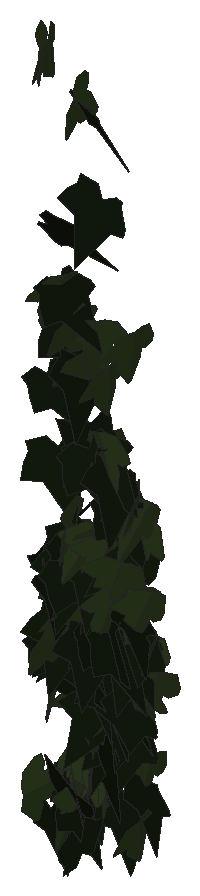
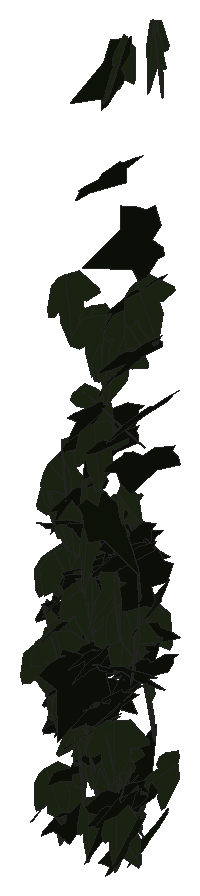
# SketchUp Ruby script. Lengths in inches.
U = 1.inch
M = Sketchup.active_model
def pt(a) = Geom::Point3d.new(a.map { |v| v * U })
def face(e, loops, mat)
  f = e.add_face(loops[0].map { |a| pt(a) })
  loops[1..].each { |l| e.add_face(l.map { |a| pt(a) }).erase! }
  f.material = f.back_material = mat if mat
  f
end
# faces: each face lists its corners as indices into pts; further lists are holes
def faces(e, pts, list, mat = nil) = list.each { |f| face(e, (f[0].is_a?(Array) ? f : [f]).map { |l| l.map { |i| pts[i] } }, mat) }
# xy, xz, yz: faces in a plane at the given z, y or x. An outline is a flat list of corners, or four numbers for a rectangle; further outlines are holes
def ring(l) = l.size == 4 ? [[l[0], l[1]], [l[2], l[1]], [l[2], l[3]], [l[0], l[3]]] : l.each_slice(2).to_a
def flat(e, list, mat, &to3) = list.each { |f| face(e, (f[0].is_a?(Array) ? f : [f]).map { |l| ring(l).map { |u, v| to3.(u, v) } }, mat) }
def xy(e, z, list, mat = nil) = flat(e, list, mat) { |x, y| [x, y, z] }
def xz(e, y, list, mat = nil) = flat(e, list, mat) { |x, z| [x, y, z] }
def yz(e, x, list, mat = nil) = flat(e, list, mat) { |y, z| [x, y, z] }
def lines(e, pts, list) = list.each { |a, b| e.add_line(pt(pts[a]), pt(pts[b])) }
# prism: a flat outline (further loops are holes) pulled along v
def prism(e, loops, v, mat = nil)
  f = face(e, loops, mat); d = Geom::Vector3d.new(v.map { |x| x * U })
  f.pushpull(f.normal.samedirection?(d) ? d.length : -d.length)
end
def box(e, o, s, mat = nil) = prism(e, [[o, [o[0] + s[0], o[1], o[2]], [o[0] + s[0], o[1] + s[1], o[2]], [o[0], o[1] + s[1], o[2]]]], [0, 0, s[2]], mat)
def at(x, y, z, deg = 0) = Geom::Transformation.translation(pt([x, y, z])) * Geom::Transformation.rotation(ORIGIN, Z_AXIS, deg.degrees)
def axes(o, x, y, z) = Geom::Transformation.new([*x, 0, *y, 0, *z, 0, *pt(o).to_a, 1])
def part(name) = M.definitions.add(name)
# library, detail: a bought-in or finely detailed component or shape, given as its bounding box
def library(name, o, s) = part(name).tap { |d| box(d.entities, o, s) }
def detail(e, o, s) = box(e.add_group.entities, o, s)
def put(e, d, t, mat = nil) = e.add_instance(d, t).tap { |i| i.material = mat if mat }
def group(e, t, mat = nil) = e.add_group.tap { |g| g.transformation = t; g.material = mat if mat }.entities
root = M.entities
M.materials.add("efeu1").color = [18, 25, 13]
M.materials.add("efeu2").color = [43, 57, 29]
c1 = part("ivyleaf_10")
p = [[0,0.5,-0.03],[-0.0625,2.02,-0.43],[-0.19,2.01,-0.46],[-0.54,1.05,-0.29],[-0.52,0.625,-0.18],[-0.83,0.76,-0.28],
  [-1.16,0.64,-0.33],[-1.15,0.33,-0.24],[-0.77,-0.39,0.02],[-0.3,-0.51,0.16],[0.04,-0.48,0.23],[-0.02,2.01,-0.4375],
  [-0.06,2.01,-0.43],[0.04,-0.49,0.23],[0.67,-0.49,0.14],[1.38,0.36,-0.2],[1.375,0.51,-0.24],[0.81,0.65,-0.19],
  [0.62,0.59,-0.15],[0.6,1.09,-0.28],[0.5,1.23,-0.31]]
faces(c1.entities,p,[[0,1,2,3,4,5,6,7,8,9,10],[11,12,0,13,14,15,16,17,18,19,20]],"efeu2")
c2 = part("ivyleaf_9")
p = [[1.54,2.16,1.25],[1.36,2.04,1.19],[-0.21,0.99,0.68],[-0.71,1.11,0.82],[-0.85,0.86,0.67],[-0.8,0.17,0.21],
  [-0.9,-0.01,0.1],[-0.67,-0.16,-0.02],[-0.08,-0.08,-0.05],[-0.03,-0.6,-0.4],[0.65,-0.88,-0.66],[0.83,-0.6,-0.49],
  [1.29,-0.42,-0.43],[1.8125,-0.07,-0.26],[1.21,0.44,0.15]]
faces(c2.entities,p,[[0,1,2,3,4,5,6,7,8,9,10,11,12,13,14]],"efeu1")
put(root,c1,axes([531.31,133.06,214.31],[0.38555,-0.60356,-0.56134],[-0.07276,0.59238,-0.68691],[0.82103,0.33592,0.20273]))
put(root,c2,axes([530.73,134.37,206.68],[0.50004,-0.69895,0.12172],[0.07493,-0.09605,-0.85939],[0.7055,0.5056,0.00501]))
put(root,c1,axes([531.26,132.02,237.24],[0.60567,-0.73019,-0.20182],[-0.01894,0.24371,-0.93861],[0.75733,0.59006,0.13793]))
put(root,c2,axes([530.76,133.04,223.34],[0.41024,-0.76261,-0.33412],[0.09273,0.41201,-0.82653],[0.82741,0.33193,0.25829]))
put(root,c1,axes([531.36,134.16,207.32],[-0.0306,-0.83738,-0.23344],[0.00435,0.23343,-0.83793],[0.8693,-0.03064,-0.00402]))
put(root,c1,axes([531.46,132.7,227.38],[-0.14113,-0.90335,0.18428],[-0.04904,-0.1788,-0.91408],[0.92065,-0.148,-0.02045]))
put(root,c2,axes([531.56,134.07,213.17],[-0.80351,-0.35056,0.01012],[0.09038,-0.23142,-0.84077],[0.33887,-0.76953,0.24824]))
put(root,c2,axes([530.95,132.92,213.08],[0.22478,-0.6736,-0.50792],[0.09563,0.54259,-0.67727],[0.8382,0.11874,0.21347]))
put(root,c1,axes([531.56,133.4,215.02],[-0.35311,-0.7704,0.22773],[-0.04685,-0.22858,-0.84594],[0.80199,-0.35255,0.05085]))
put(root,c1,axes([531.44,133.86,206.71],[0.07082,-0.76777,0.36554],[0.05311,-0.36209,-0.77083],[0.84869,0.08672,0.01774]))
put(root,c2,axes([530.98,132.84,206.17],[0.32279,-0.7566,0.18108],[0.0695,-0.16722,-0.82258],[0.77486,0.33018,-0.00166]))
put(root,c1,axes([531.56,134.09,210.61],[-0.51691,-0.71114,-0.02205],[0.06157,-0.01756,-0.8771],[0.70881,-0.51708,0.06011]))
put(root,c2,axes([531.27,134.17,207.89],[0.36615,-0.5321,-0.55869],[-0.27836,0.48566,-0.64497],[0.71957,0.45862,0.03479]))
put(root,c1,axes([531.55,131.9,237.3],[0.26569,-0.83161,-0.43011],[0.00191,0.44757,-0.8642],[0.93626,0.23508,0.12382]))
put(root,c1,axes([531.6,132.23,211.63],[0.48606,-0.70274,-0.28183],[-0.12268,0.25739,-0.85336],[0.74714,0.49943,0.04323]))
put(root,c1,axes([531.4,131.21,207.92],[0.0765,-0.10269,-0.94407],[0.27818,0.908,-0.07622],[0.90798,-0.26954,0.1029]))
put(root,c1,axes([531.65,133.45,214.53],[-0.57947,-0.65111,-0.09346],[0.05323,0.07773,-0.87155],[0.65563,-0.58179,-0.01185]))
put(root,c1,axes([531.52,134.33,210.18],[0.48114,-0.71154,0.07292],[0.07994,-0.03383,-0.85765],[0.71078,0.48545,0.0471]))
put(root,c2,axes([531.17,132.9375,214.83],[0.05217,-0.67786,0.55598],[0.18506,-0.5359,-0.67074],[0.85695,0.15699,0.111]))
put(root,c1,axes([531.84,133.61,215.99],[0.38725,-0.53266,-0.59096],[-0.25962,0.53666,-0.65385],[0.75204,0.45956,0.07859]))
put(root,c1,axes([531.82,132.46,215.96],[0.47407,-0.73454,-0.50008],[-0.14605,0.49468,-0.86507],[0.87653,0.4797,0.12632]))
put(root,c1,axes([531.79,132.96,214.22],[-0.43697,-0.74668,-0.15234],[0.05657,0.14334,-0.86483],[0.75996,-0.44001,-0.02322]))
put(root,c1,axes([531.94,133.71,215.85],[-0.01054,0.17131,0.86807],[-0.36442,0.79024,-0.16038],[-0.80628,-0.35941,0.06114]))
put(root,c2,axes([531.38,133.27,225.4],[0.14211,-0.86458,-0.27161],[0.08904,0.28692,-0.86673],[0.90186,0.10791,0.12837]))
put(root,c2,axes([531.2,132.65,216.01],[0.23828,-0.06865,0.85647],[0.8442,0.18414,-0.22011],[-0.15993,0.86972,0.11421]))
put(root,c2,axes([531.78,132.79,214.02],[-0.5604,-0.68176,-0.20575],[0.1371,0.15363,-0.88249],[0.69881,-0.57687,0.00814]))
put(root,c2,axes([531.1875,132.64,229.65],[0.88444,-0.09046,0.31445],[0.31285,-0.03169,-0.88905],[0.09585,0.93814,0.00029]))
put(root,c2,axes([531.54,132.54,220.9],[-0.14463,-0.80789,-0.42978],[0.15271,0.4077,-0.81778],[0.90226,-0.19851,0.06952]))
put(root,c1,axes([531.9375,131.45,213.97],[-0.20913,-0.61059,-0.74498],[0.20884,0.71546,-0.64502],[0.94032,-0.2947,-0.02244]))
put(root,c2,axes([531.66,133.3,217.22],[0.03492,-0.84123,-0.33092],[0.06151,0.33261,-0.83904],[0.90188,0.00988,0.07004]))
put(root,c1,axes([532.0625,133.6,215.53],[-0.36583,-0.70571,0.40923],[0.10244,-0.48469,-0.74425],[0.80932,-0.25765,0.27918]))
put(root,c2,axes([531.62,132.61,227.42],[0.36174,-0.74749,-0.4514],[-0.0321,0.47689,-0.81542],[0.87263,0.32741,0.15713]))
put(root,c1,axes([532.06,132.68,226],[-0.23724,-0.75455,-0.51758],[0.14702,0.49632,-0.79094],[0.90312,-0.27901,-0.0072]))
put(root,c2,axes([531.83,133.65,207.43],[-0.05794,-0.83191,-0.14877],[0.00108,0.14905,-0.83388],[0.84511,-0.05722,-0.00913]))
put(root,c2,axes([532.51,133.66,218.99],[-0.46241,0.71726,-0.27291],[0.01946,-0.30756,-0.84131],[-0.76718,-0.44013,0.14315]))
put(root,c1,axes([532.75,132.52,214.16],[0.23584,0.0086,-0.88225],[-0.84813,0.25387,-0.22425],[0.24313,0.87723,0.07355]))
put(root,c2,axes([531.89,133.55,207.86],[-0.03088,-0.80519,-0.39924],[0.02736,0.39845,-0.80571],[0.89832,-0.03982,0.01082]))
put(root,c1,axes([532.07,132.8125,208.02],[-0.38647,0.73817,-0.21038],[0.09403,-0.18824,-0.83321],[-0.76179,-0.39772,0.00389]))
put(root,c2,axes([531.84,133.35,211.45],[0.14551,-0.82173,0.2304],[0.15707,-0.20395,-0.82658],[0.83884,0.18073,0.11481]))
put(root,c2,axes([532.32,132.33,207.1875],[0.67125,-0.44023,0.40048],[-0.33428,0.22055,0.80274],[-0.49239,-0.74988,0.00098]))
put(root,c2,axes([532.13,132.49,217.6],[0.18109,-0.52398,-0.70922],[-0.2471,0.66485,-0.5543],[0.84645,0.30619,-0.01009]))
put(root,c2,axes([532.22,134.11,211.43],[-0.20707,-0.85297,0.01207],[0.00344,-0.01326,-0.87772],[0.85305,-0.20699,0.00647]))
put(root,c2,axes([532.39,132.67,216.77],[-0.55726,-0.73513,-0.12476],[0.05694,0.11335,-0.92218],[0.74346,-0.55969,-0.02289]))
put(root,c1,axes([532.5,134.25,207.3],[0.07736,-0.82771,-0.20258],[0.03896,0.20663,-0.8294],[0.85125,0.06577,0.05637]))
put(root,c2,axes([532.16,134.15,213.53],[0.16524,-0.85872,0.01341],[-0.00032,-0.01372,-0.87447],[0.85882,0.16522,-0.00291]))
put(root,c1,axes([532.5625,134.65,209.65],[0.42235,-0.71185,-0.2197],[-0.02377,0.23955,-0.82185],[0.74461,0.41142,0.09839]))
put(root,c1,axes([532.58,132.61,224.8125],[-0.31543,-0.8219,-0.31637],[0.10356,0.29911,-0.88029],[0.87458,-0.33184,-0.00987]))
put(root,c1,axes([532.5,132.96,208.97],[0.57246,0.61048,-0.20411],[-0.11839,-0.16864,-0.83642],[-0.63272,0.58389,-0.02817]))
put(root,c1,axes([532.43,132.39,218.8125],[0.29086,-0.66861,0.59019],[0.30293,-0.5098,-0.72684],[0.8388,0.41596,0.05785]))
put(root,c1,axes([532.51,132.35,207.46],[0.05009,-0.70202,0.61785],[0.24348,-0.58761,-0.6874],[0.90293,0.1974,0.15108]))
put(root,c1,axes([532.72,134.07,217.875],[0.16388,-0.73005,-0.46171],[-0.03906,0.4632,-0.74628],[0.86292,0.15962,0.05391]))
put(root,c1,axes([533,133.49,216.74],[-0.43486,-0.4296,0.66141],[-0.34127,-0.57841,-0.60007],[0.71101,-0.54037,0.11649]))
put(root,c1,axes([532.74,133.21,225.81],[-0.77789,-0.48788,-0.031],[0.04364,-0.01127,-0.91764],[0.48691,-0.77842,0.03272]))
put(root,c1,axes([532.74,133.75,216.09],[0.19134,-0.81308,-0.32498],[-0.02485,0.32747,-0.83395],[0.87527,0.18705,0.04737]))
put(root,c2,axes([532.38,132.71,224.16],[0.08598,-0.89241,0.28531],[0.00142,-0.28638,-0.8962],[0.93691,0.08233,-0.02483]))
put(root,c1,axes([532.9,133.5,208.9375],[-0.46583,-0.6684,0.35346],[-0.08055,-0.36892,-0.80381],[0.7518,-0.45369,0.13288]))
put(root,c2,axes([533.43,132.08,221.72],[-0.28187,0.57149,0.64541],[-0.54893,0.40459,-0.59799],[-0.6647,-0.57647,0.22015]))
put(root,c2,axes([532.81,134.16,212.62],[0.49202,0.72434,-0.01563],[-0.02514,-0.00181,-0.87542],[-0.72407,0.49226,0.01978]))
put(root,c2,axes([532.47,132.32,207.32],[0.31689,-0.74652,-0.26021],[-0.06764,0.25371,-0.81023],[0.78767,0.32212,0.03511]))
put(root,c1,axes([532.98,133.82,209.83],[0.02079,-0.8764,-0.02765],[-0.00126,0.02762,-0.87664],[0.87683,0.02082,-0.0006]))
put(root,c1,axes([532.78,133.89,210.15],[0.37943,-0.75077,0.22454],[0.21086,-0.14246,-0.83264],[0.75473,0.41724,0.11974]))
put(root,c2,axes([532.49,131.89,216.96],[0.37475,-0.6045,-0.70261],[-0.04981,0.74364,-0.66637],[0.92553,0.28479,0.24863]))
put(root,c1,axes([532.72,133.05,208.88],[0.74599,0.41479,0.1404],[0.12893,0.05701,-0.85346],[-0.4185,0.75694,-0.01266]))
put(root,c1,axes([533.07,132.53,218.01],[-0.30655,-0.82735,-0.13894],[0.02839,0.13762,-0.88207],[0.83846,-0.30715,-0.02094]))
put(root,c1,axes([533.09,132.4,218.02],[-0.23874,-0.63954,0.58],[-0.01364,-0.59889,-0.666],[0.86326,-0.18634,0.14988]))
put(root,c1,axes([533.14,133.8,215.49],[-0.4578,-0.74486,0.14939],[-0.0223,-0.16117,-0.87192],[0.75936,-0.45378,0.06446]))
put(root,c2,axes([533.44,131.48,206.12],[-0.75804,0.34514,-0.36247],[-0.33782,0.13257,0.83272],[0.3693,0.82972,0.01772]))
put(root,c1,axes([533.11,133.16,221.39],[-0.20642,-0.8997,-0.06173],[0.00489,0.06221,-0.92303],[0.9018,-0.20627,-0.00913]))
put(root,c2,axes([532.68,133.49,213.23],[0.05114,-0.86786,-0.22976],[0.03693,0.23197,-0.86799],[0.897,0.03993,0.04883]))
put(root,c2,axes([533.04,133.79,216.23],[-0.573,-0.68403,0.03057],[0.02745,-0.06278,-0.89021],[0.68416,-0.57038,0.06132]))
put(root,c2,axes([532.97,134.64,209.03],[-0.30943,-0.78496,0.11855],[0.00926,-0.1308,-0.84188],[0.79381,-0.30446,0.05603]))
put(root,c2,axes([532.97,132.76,213.75],[-0.31182,-0.81495,-0.1063],[0.01122,0.10946,-0.87211],[0.82178,-0.31073,-0.02843]))
put(root,c2,axes([532.6875,133.4,217.67],[-0.32571,-0.45171,-0.70705],[0.64127,0.35507,-0.52225],[0.54105,-0.69277,0.19335]))
put(root,c1,axes([533.17,131.48,235.84],[0.12046,-0.59248,-0.75944],[0.05336,0.76828,-0.59091],[0.96173,0.03158,0.1279]))
put(root,c2,axes([532.78,132.79,221.13],[0.15257,-0.82717,-0.39116],[0.01296,0.39847,-0.83759],[0.91491,0.1323,0.07709]))
put(root,c2,axes([532.93,133.47,215.98],[-0.50318,-0.15655,-0.70433],[0.71229,0.02913,-0.51535],[0.11504,-0.86512,0.1101]))
put(root,c2,axes([533.19,133.69,216.42],[-0.43247,-0.77497,0.13157],[-0.03339,-0.13192,-0.88679],[0.78535,-0.43236,0.03475]))
put(root,c2,axes([533.35,132.79,211.18],[-0.61755,-0.60535,0.08134],[-0.03064,-0.08481,-0.86388],[0.61002,-0.61708,0.03894]))
put(root,c2,axes([533.2,133.85,209.77],[-0.41077,-0.60773,0.49349],[0.00037,-0.55744,-0.68619],[0.78286,-0.31861,0.25926]))
put(root,c1,axes([533.0625,132.6,209.64],[-0.2862,0.50806,-0.64258],[0.18225,-0.62412,-0.57463],[-0.79863,-0.32449,0.09914]))
put(root,c1,axes([533.41,133.18,219.125],[0.22177,-0.84703,-0.28223],[-0.04335,0.28025,-0.87514],[0.89176,0.22427,0.02764]))
put(root,c1,axes([533.38,132.83,207.36],[0.51462,-0.67349,-0.09226],[-0.05536,0.0738,-0.84759],[0.67752,0.51759,0.00081]))
put(root,c1,axes([533.56,132.78,217.65],[-0.37679,-0.72651,0.42423],[-0.07,-0.43615,-0.80909],[0.83838,-0.36292,0.1231]))
put(root,c2,axes([532.94,134.32,211.74],[0.45595,-0.72125,-0.16298],[0.00632,0.19526,-0.84646],[0.73941,0.44308,0.10773]))
put(root,c2,axes([533.31,132.68,231.32],[-0.27865,-0.85434,0.28727],[0.00457,-0.30202,-0.89377],[0.90133,-0.26259,0.09334]))
put(root,c2,axes([533.37,132.5,217.25],[-0.55457,-0.67028,-0.3031],[0.20834,0.22093,-0.86976],[0.70551,-0.59212,0.01859]))
put(root,c2,axes([533.38,133.875,213.02],[-0.26394,-0.84156,-0.04058],[0.01823,0.03681,-0.88195],[0.84234,-0.26449,0.00638]))
put(root,c2,axes([533.3,133.43,215.59],[-0.05872,-0.86578,0.26803],[0.03366,-0.27049,-0.86636],[0.9057,-0.04608,0.04958]))
put(root,c2,axes([533.05,131.99,235.45],[0.80173,-0.54579,0.07032],[0.05191,-0.0487,-0.96981],[0.54785,0.80333,-0.01102]))
put(root,c2,axes([533.59,132.94,210.36],[-0.71293,-0.22437,-0.44965],[0.46846,-0.01429,-0.73562],[0.18185,-0.84276,0.13218]))
put(root,c1,axes([533.55,132.84,210.39],[-0.21265,-0.59928,-0.74567],[0.28399,0.68989,-0.63544],[0.91352,-0.35397,0.02396]))
put(root,c2,axes([533.4375,133.19,212.11],[-0.16998,-0.82115,-0.27496],[0.04003,0.27246,-0.83842],[0.86503,-0.17396,-0.01523]))
put(root,c2,axes([533.41,134.09,206.84],[-0.07366,-0.85929,-0.13451],[0.01593,0.13363,-0.86243],[0.8696,-0.07523,0.00441]))
put(root,c2,axes([533.18,134.05,211.1875],[0.4856,-0.70894,0.17463],[0.12742,-0.12422,-0.85862],[0.71892,0.50087,0.03423]))
put(root,c1,axes([533.83,134.78,208.28],[-0.14618,-0.80825,0.19938],[-0.00992,-0.20073,-0.82098],[0.83242,-0.14433,0.02523]))
put(root,c1,axes([534.01,133.68,213.64],[-0.60897,-0.6118,0.19593],[-0.02114,-0.25074,-0.84865],[0.64206,-0.58853,0.15788]))
put(root,c2,axes([533.48,133.33,211.4],[0.25542,-0.79521,0.25974],[0.09082,-0.24362,-0.83515],[0.83162,0.27084,0.01143]))
put(root,c2,axes([533.47,131.94,221.79],[0.13484,-0.69,-0.66873],[0.19886,0.6807,-0.66226],[0.94008,-0.04502,0.23601]))
put(root,c1,axes([533.85,132.19,222.07],[-0.85604,0.16176,-0.25789],[0.20563,-0.2603,-0.84583],[-0.22448,-0.85531,0.20864]))
put(root,c1,axes([534.03,134.14,213.32],[-0.66983,-0.53387,0.18484],[0.065,-0.35761,-0.79734],[0.56121,-0.59578,0.31296]))
put(root,c1,axes([534.03,133.73,210.875],[0.05796,-0.74159,0.49205],[0.07603,-0.48717,-0.74318],[0.88673,0.09025,0.03156]))
put(root,c2,axes([533.64,133.2,219.15],[0.2604,-0.79471,-0.38438],[-0.0211,0.39504,-0.83104],[0.88254,0.24394,0.09355]))
put(root,c2,axes([533.4,132.18,214.64],[-0.02786,-0.27695,-0.87625],[0.85197,0.32083,-0.12849],[0.34448,-0.81588,0.24692]))
put(root,c2,axes([534.08,133.37,210.08],[-0.50134,-0.70507,-0.10785],[0.04583,0.09971,-0.86491],[0.7118,-0.50303,-0.02027]))
put(root,c1,axes([534.1875,131.93,225.1],[-0.05326,-0.93016,-0.17136],[0.04175,0.16915,-0.93115],[0.94489,-0.05991,0.03149]))
put(root,c1,axes([534.28,132.19,216.11],[-0.16439,-0.83355,0.36866],[0.047,-0.38186,-0.84244],[0.91022,-0.13083,0.11008]))
put(root,c2,axes([534.5,133.45,217.62],[-0.79444,-0.38878,0.17348],[-0.0207,-0.33158,-0.83786],[0.42523,-0.74249,0.28333]))
put(root,c1,axes([534.375,133.54,211.87],[-0.87418,0.07531,0.0181],[-0.01792,0.00288,-0.87741],[-0.07535,-0.87436,-0.00133]))
put(root,c2,axes([533.86,132.17,209.89],[-0.26962,-0.00969,-0.84737],[0.84438,0.0723,-0.2695],[0.07183,-0.88629,-0.01272]))
put(root,c1,axes([534.68,131.99,217.44],[-0.6923,-0.54025,0.31172],[-0.23448,-0.20611,-0.87799],[0.57798,-0.73073,0.01719]))
put(root,c2,axes([534.03,133.5,213.93],[0.2033,-0.84803,-0.23704],[-0.00974,0.24109,-0.87089],[0.88048,0.19848,0.04509]))
put(root,c2,axes([534.27,133.3125,211.28],[-0.20239,-0.82196,0.17649],[-0.02879,-0.17465,-0.84641],[0.84021,-0.20398,0.01351]))
put(root,c2,axes([534.04,134.29,207.46],[0.235,-0.80998,0.18846],[0.05622,-0.17992,-0.84337],[0.82971,0.2416,0.00377]))
put(root,c1,axes([534.64,133.21,215.875],[-0.38643,-0.69108,0.39779],[-0.06913,-0.41134,-0.78178],[0.79439,-0.37197,0.12547]))
put(root,c2,axes([534.28,132.41,220.83],[-0.03895,-0.91158,0.17875],[-0.00492,-0.17871,-0.91241],[0.92893,-0.03917,0.00266]))
put(root,c1,axes([534.62,133.47,218.43],[0.87156,-0.13694,-0.20885],[-0.19159,0.11975,-0.87803],[0.16021,0.8882,0.08618]))
put(root,c1,axes([534.67,133.01,206.73],[-0.03703,-0.83015,-0.259],[-0.00166,0.2593,-0.83088],[0.86961,-0.03485,-0.01261]))
put(root,c2,axes([534.31,132.1,214.53],[0.38062,-0.84013,-0.35561],[-0.08147,0.35248,-0.91993],[0.90865,0.38352,0.06648]))
put(root,c1,axes([534.93,133.71,212.37],[-0.50534,-0.70939,0.2274],[-0.12643,-0.18913,-0.87095],[0.73414,-0.52087,0.00654]))
put(root,c1,axes([534.83,132.58,226.41],[-0.16313,-0.93617,-0.03922],[0.00945,0.03816,-0.95027],[0.93694,-0.16338,0.00276]))
put(root,c2,axes([534.29,133.26,215.0625],[0.26512,-0.82556,0.2728],[0.11551,-0.24923,-0.86649],[0.86176,0.28739,0.03221]))
put(root,c1,axes([534.84,132.69,219.94],[0.36396,-0.77059,-0.31438],[-0.05794,0.31884,-0.84858],[0.83023,0.36006,0.0786]))
put(root,c1,axes([534.94,133.18,215.75],[-0.30013,-0.76011,0.36353],[-0.02612,-0.37733,-0.81052],[0.84216,-0.28259,0.10442]))
put(root,c2,axes([534.74,132.87,214.21],[-0.36394,-0.83749,-0.02495],[0.00913,0.02324,-0.91315],[0.83782,-0.36405,-0.00088]))
put(root,c1,axes([534.85,133.57,213.77],[0.48274,-0.73974,0.02869],[0.01692,-0.02322,-0.88332],[0.74011,0.48304,0.00148]))
put(root,c1,axes([534.92,133.04,219.32],[-0.16096,-0.71974,0.56052],[0.08239,-0.57832,-0.71894],[0.90853,-0.07507,0.16451]))
